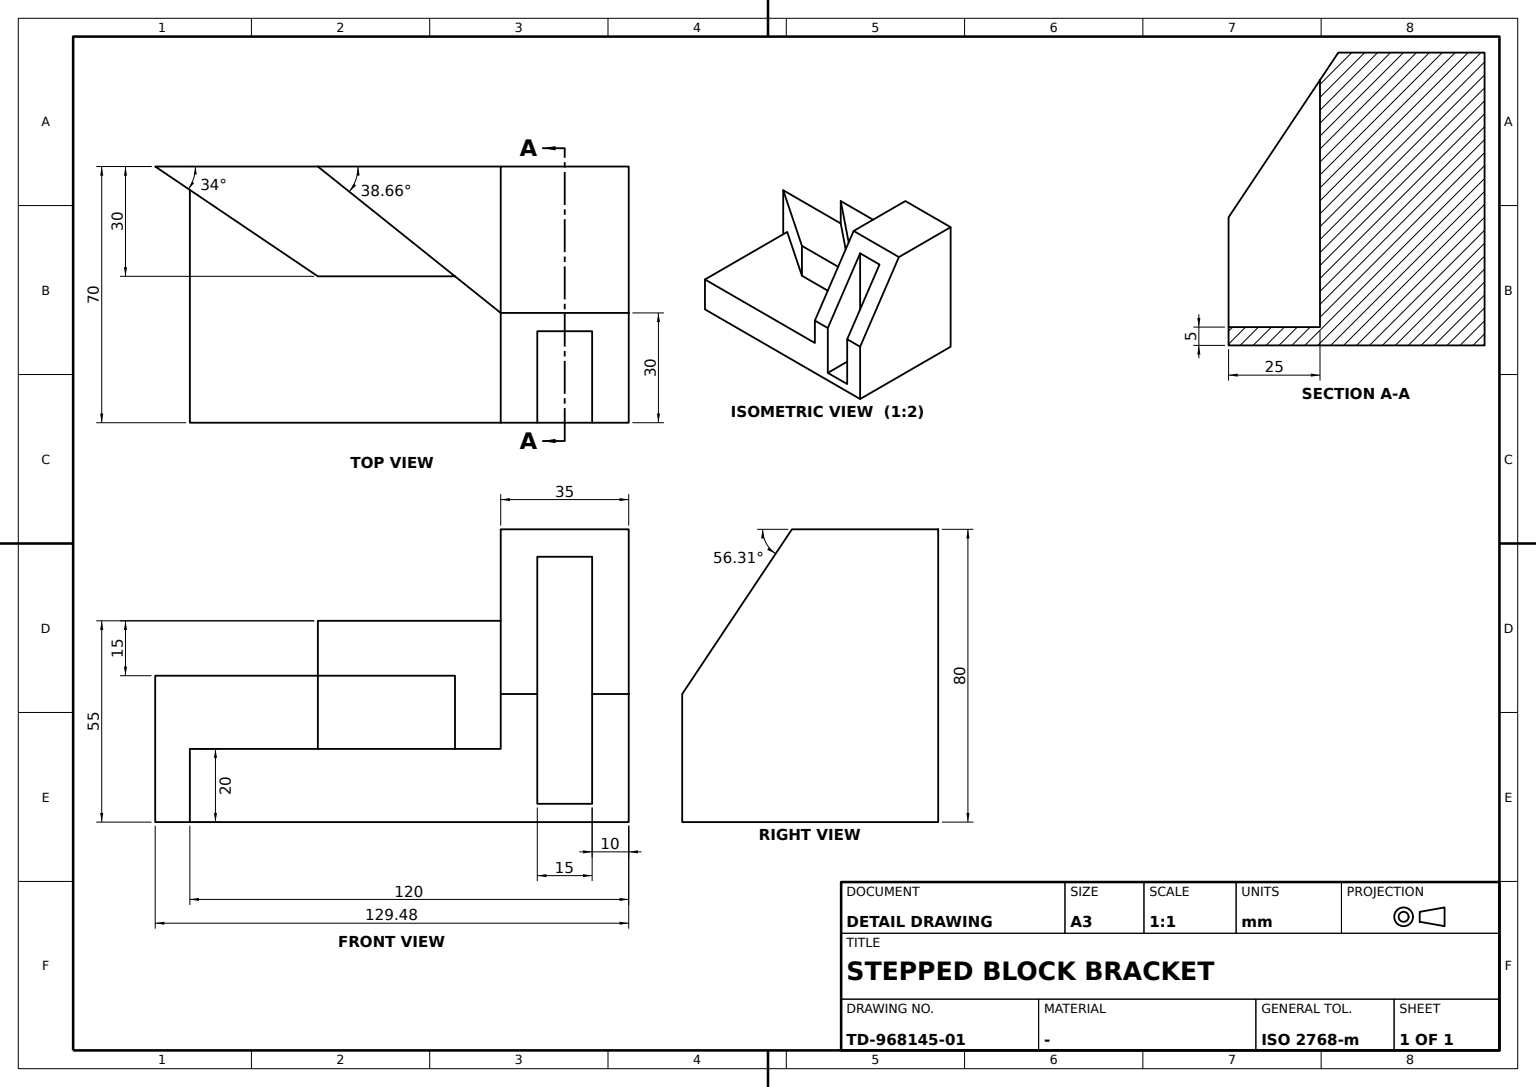
ISO-10303-21;
HEADER;
FILE_DESCRIPTION((''),'2;1');
FILE_NAME('','',(''),(''),'','','');
FILE_SCHEMA(('AUTOMOTIVE_DESIGN'));
ENDSEC;
DATA;
#1=APPLICATION_CONTEXT('');
#2=PRODUCT_CONTEXT('',#1,'mechanical');
#3=PRODUCT('','','',(#2));
#4=PRODUCT_DEFINITION_FORMATION('','',#3);
#5=PRODUCT_DEFINITION_CONTEXT('',#1,'design');
#6=PRODUCT_DEFINITION('','',#4,#5);
#7=PRODUCT_DEFINITION_SHAPE('','',#6);
#8=(LENGTH_UNIT()NAMED_UNIT(*)SI_UNIT(.MILLI.,.METRE.));
#9=(NAMED_UNIT(*)PLANE_ANGLE_UNIT()SI_UNIT($,.RADIAN.));
#10=(NAMED_UNIT(*)SI_UNIT($,.STERADIAN.)SOLID_ANGLE_UNIT());
#11=UNCERTAINTY_MEASURE_WITH_UNIT(LENGTH_MEASURE(0.005),#8,'distance_accuracy_value','');
#12=(GEOMETRIC_REPRESENTATION_CONTEXT(3)GLOBAL_UNCERTAINTY_ASSIGNED_CONTEXT((#11))GLOBAL_UNIT_ASSIGNED_CONTEXT((#8,#9,#10))REPRESENTATION_CONTEXT('',''));
#13=CARTESIAN_POINT('',(35.,50.,5.));
#14=VERTEX_POINT('',#13);
#15=CARTESIAN_POINT('',(35.,50.,35.));
#16=VERTEX_POINT('',#15);
#17=DIRECTION('',(0.,0.,1.));
#18=VECTOR('',#17,1000.);
#19=LINE('',#13,#18);
#20=EDGE_CURVE('',#14,#16,#19,.T.);
#21=ORIENTED_EDGE('',*,*,#20,.F.);
#22=CARTESIAN_POINT('',(35.,35.,5.));
#23=VERTEX_POINT('',#22);
#24=DIRECTION('',(0.,1.,0.));
#25=VECTOR('',#24,1000.);
#26=LINE('',#22,#25);
#27=EDGE_CURVE('',#23,#14,#26,.T.);
#28=ORIENTED_EDGE('',*,*,#27,.F.);
#29=CARTESIAN_POINT('',(35.,35.,35.));
#30=VERTEX_POINT('',#29);
#31=LINE('',#22,#18);
#32=EDGE_CURVE('',#23,#30,#31,.T.);
#33=ORIENTED_EDGE('',*,*,#32,.T.);
#34=CARTESIAN_POINT('',(35.,25.,35.));
#35=VERTEX_POINT('',#34);
#36=CARTESIAN_POINT('',(35.,85.,35.));
#37=DIRECTION('',(0.,-1.,0.));
#38=VECTOR('',#37,1000.);
#39=LINE('',#36,#38);
#40=EDGE_CURVE('',#30,#35,#39,.T.);
#41=ORIENTED_EDGE('',*,*,#40,.T.);
#42=CARTESIAN_POINT('',(35.,25.,20.));
#43=VERTEX_POINT('',#42);
#44=CARTESIAN_POINT('',(35.,25.,80.));
#45=DIRECTION('',(0.,0.,-1.));
#46=VECTOR('',#45,1000.);
#47=LINE('',#44,#46);
#48=EDGE_CURVE('',#35,#43,#47,.T.);
#49=ORIENTED_EDGE('',*,*,#48,.T.);
#50=CARTESIAN_POINT('',(35.,-60.,20.));
#51=VERTEX_POINT('',#50);
#52=LINE('',#50,#25);
#53=EDGE_CURVE('',#51,#43,#52,.T.);
#54=ORIENTED_EDGE('',*,*,#53,.F.);
#55=CARTESIAN_POINT('',(35.,-60.,0.));
#56=VERTEX_POINT('',#55);
#57=LINE('',#50,#46);
#58=EDGE_CURVE('',#51,#56,#57,.T.);
#59=ORIENTED_EDGE('',*,*,#58,.T.);
#60=CARTESIAN_POINT('',(35.,60.,0.));
#61=VERTEX_POINT('',#60);
#62=LINE('',#55,#25);
#63=EDGE_CURVE('',#56,#61,#62,.T.);
#64=ORIENTED_EDGE('',*,*,#63,.T.);
#65=CARTESIAN_POINT('',(35.,60.,35.));
#66=VERTEX_POINT('',#65);
#67=CARTESIAN_POINT('',(35.,60.,20.));
#68=LINE('',#67,#46);
#69=EDGE_CURVE('',#66,#61,#68,.T.);
#70=ORIENTED_EDGE('',*,*,#69,.F.);
#71=EDGE_CURVE('',#66,#16,#39,.T.);
#72=ORIENTED_EDGE('',*,*,#71,.T.);
#73=EDGE_LOOP('',(#21,#28,#33,#41,#49,#54,#59,#64,#70,#72));
#74=FACE_BOUND('',#73,.T.);
#75=DIRECTION('',(-1.,0.,0.));
#76=AXIS2_PLACEMENT_3D('',#50,#75,#37);
#77=PLANE('',#76);
#78=ADVANCED_FACE('',(#74),#77,.F.);
#79=CARTESIAN_POINT('',(5.,60.,80.));
#80=VERTEX_POINT('',#79);
#81=CARTESIAN_POINT('',(41.923077,60.,24.615385));
#82=DIRECTION('',(0.554700196,0.,-0.832050294));
#83=VECTOR('',#82,1000.);
#84=LINE('',#81,#83);
#85=EDGE_CURVE('',#80,#66,#84,.T.);
#86=ORIENTED_EDGE('',*,*,#85,.F.);
#87=CARTESIAN_POINT('',(5.,25.,80.));
#88=VERTEX_POINT('',#87);
#89=CARTESIAN_POINT('',(5.,85.,80.));
#90=LINE('',#89,#38);
#91=EDGE_CURVE('',#80,#88,#90,.T.);
#92=ORIENTED_EDGE('',*,*,#91,.T.);
#93=LINE('',#87,#83);
#94=EDGE_CURVE('',#88,#35,#93,.T.);
#95=ORIENTED_EDGE('',*,*,#94,.T.);
#96=ORIENTED_EDGE('',*,*,#40,.F.);
#97=CARTESIAN_POINT('',(10.,35.,72.5));
#98=VERTEX_POINT('',#97);
#99=CARTESIAN_POINT('',(5.,35.,80.));
#100=DIRECTION('',(-0.554700196,0.,0.832050294));
#101=VECTOR('',#100,1000.);
#102=LINE('',#99,#101);
#103=EDGE_CURVE('',#30,#98,#102,.T.);
#104=ORIENTED_EDGE('',*,*,#103,.T.);
#105=CARTESIAN_POINT('',(10.,50.,72.5));
#106=VERTEX_POINT('',#105);
#107=CARTESIAN_POINT('',(10.,85.,72.5));
#108=LINE('',#107,#25);
#109=EDGE_CURVE('',#98,#106,#108,.T.);
#110=ORIENTED_EDGE('',*,*,#109,.T.);
#111=CARTESIAN_POINT('',(5.,50.,80.));
#112=LINE('',#111,#83);
#113=EDGE_CURVE('',#106,#16,#112,.T.);
#114=ORIENTED_EDGE('',*,*,#113,.T.);
#115=ORIENTED_EDGE('',*,*,#71,.F.);
#116=EDGE_LOOP('',(#86,#92,#95,#96,#104,#110,#114,#115));
#117=FACE_BOUND('',#116,.T.);
#118=DIRECTION('',(-0.832050294,0.,-0.554700196));
#119=AXIS2_PLACEMENT_3D('',#89,#118,#100);
#120=PLANE('',#119);
#121=ADVANCED_FACE('',(#117),#120,.F.);
#122=CARTESIAN_POINT('',(10.,35.,5.));
#123=VERTEX_POINT('',#122);
#124=VECTOR('',#75,1000.);
#125=LINE('',#122,#124);
#126=EDGE_CURVE('',#23,#123,#125,.T.);
#127=ORIENTED_EDGE('',*,*,#126,.T.);
#128=LINE('',#122,#46);
#129=EDGE_CURVE('',#98,#123,#128,.T.);
#130=ORIENTED_EDGE('',*,*,#129,.F.);
#131=ORIENTED_EDGE('',*,*,#103,.F.);
#132=ORIENTED_EDGE('',*,*,#32,.F.);
#133=EDGE_LOOP('',(#127,#130,#131,#132));
#134=FACE_BOUND('',#133,.T.);
#135=AXIS2_PLACEMENT_3D('',#122,#37,#45);
#136=PLANE('',#135);
#137=ADVANCED_FACE('',(#134),#136,.F.);
#138=CARTESIAN_POINT('',(-35.,-25.,40.));
#139=VERTEX_POINT('',#138);
#140=CARTESIAN_POINT('',(-5.,12.5,40.));
#141=VERTEX_POINT('',#140);
#142=DIRECTION('',(0.624695048,0.780868809,0.));
#143=VECTOR('',#142,1000.);
#144=LINE('',#138,#143);
#145=EDGE_CURVE('',#139,#141,#144,.T.);
#146=ORIENTED_EDGE('',*,*,#145,.F.);
#147=CARTESIAN_POINT('',(-35.,-69.476829,40.));
#148=VERTEX_POINT('',#147);
#149=LINE('',#147,#25);
#150=EDGE_CURVE('',#148,#139,#149,.T.);
#151=ORIENTED_EDGE('',*,*,#150,.F.);
#152=CARTESIAN_POINT('',(-5.,-25.,40.));
#153=VERTEX_POINT('',#152);
#154=DIRECTION('',(-0.559192903,-0.829037573,0.));
#155=VECTOR('',#154,1000.);
#156=LINE('',#152,#155);
#157=EDGE_CURVE('',#153,#148,#156,.T.);
#158=ORIENTED_EDGE('',*,*,#157,.F.);
#159=LINE('',#140,#38);
#160=EDGE_CURVE('',#141,#153,#159,.T.);
#161=ORIENTED_EDGE('',*,*,#160,.F.);
#162=EDGE_LOOP('',(#146,#151,#158,#161));
#163=FACE_BOUND('',#162,.T.);
#164=CARTESIAN_POINT('',(0.,0.,40.));
#165=AXIS2_PLACEMENT_3D('',#164,#45,#75);
#166=PLANE('',#165);
#167=ADVANCED_FACE('',(#163),#166,.F.);
#168=CARTESIAN_POINT('',(-35.,25.,80.));
#169=VERTEX_POINT('',#168);
#170=DIRECTION('',(1.,0.,0.));
#171=VECTOR('',#170,1000.);
#172=LINE('',#168,#171);
#173=EDGE_CURVE('',#169,#88,#172,.T.);
#174=ORIENTED_EDGE('',*,*,#173,.F.);
#175=CARTESIAN_POINT('',(-35.,25.,55.));
#176=VERTEX_POINT('',#175);
#177=LINE('',#168,#46);
#178=EDGE_CURVE('',#169,#176,#177,.T.);
#179=ORIENTED_EDGE('',*,*,#178,.T.);
#180=CARTESIAN_POINT('',(5.,25.,55.));
#181=VERTEX_POINT('',#180);
#182=LINE('',#180,#124);
#183=EDGE_CURVE('',#181,#176,#182,.T.);
#184=ORIENTED_EDGE('',*,*,#183,.F.);
#185=CARTESIAN_POINT('',(5.,25.,20.));
#186=VERTEX_POINT('',#185);
#187=LINE('',#180,#46);
#188=EDGE_CURVE('',#181,#186,#187,.T.);
#189=ORIENTED_EDGE('',*,*,#188,.T.);
#190=CARTESIAN_POINT('',(-35.,25.,20.));
#191=LINE('',#190,#171);
#192=EDGE_CURVE('',#186,#43,#191,.T.);
#193=ORIENTED_EDGE('',*,*,#192,.T.);
#194=ORIENTED_EDGE('',*,*,#48,.F.);
#195=ORIENTED_EDGE('',*,*,#94,.F.);
#196=EDGE_LOOP('',(#174,#179,#184,#189,#193,#194,#195));
#197=FACE_BOUND('',#196,.T.);
#198=AXIS2_PLACEMENT_3D('',#168,#24,#75);
#199=PLANE('',#198);
#200=ADVANCED_FACE('',(#197),#199,.F.);
#201=CARTESIAN_POINT('',(-35.,60.,0.));
#202=VERTEX_POINT('',#201);
#203=LINE('',#60,#124);
#204=EDGE_CURVE('',#61,#202,#203,.T.);
#205=ORIENTED_EDGE('',*,*,#204,.F.);
#206=ORIENTED_EDGE('',*,*,#63,.F.);
#207=CARTESIAN_POINT('',(-28.607798,-60.,0.));
#208=VERTEX_POINT('',#207);
#209=CARTESIAN_POINT('',(-35.,-60.,0.));
#210=LINE('',#209,#171);
#211=EDGE_CURVE('',#208,#56,#210,.T.);
#212=ORIENTED_EDGE('',*,*,#211,.F.);
#213=CARTESIAN_POINT('',(-35.,-69.476829,0.));
#214=VERTEX_POINT('',#213);
#215=CARTESIAN_POINT('',(-5.,-25.,0.));
#216=LINE('',#215,#155);
#217=EDGE_CURVE('',#208,#214,#216,.T.);
#218=ORIENTED_EDGE('',*,*,#217,.T.);
#219=LINE('',#201,#38);
#220=EDGE_CURVE('',#202,#214,#219,.T.);
#221=ORIENTED_EDGE('',*,*,#220,.F.);
#222=EDGE_LOOP('',(#205,#206,#212,#218,#221));
#223=FACE_BOUND('',#222,.T.);
#224=CARTESIAN_POINT('',(0.,0.,0.));
#225=AXIS2_PLACEMENT_3D('',#224,#17,#170);
#226=PLANE('',#225);
#227=ADVANCED_FACE('',(#223),#226,.F.);
#228=ORIENTED_EDGE('',*,*,#150,.T.);
#229=CARTESIAN_POINT('',(-35.,-25.,55.));
#230=VERTEX_POINT('',#229);
#231=LINE('',#229,#46);
#232=EDGE_CURVE('',#230,#139,#231,.T.);
#233=ORIENTED_EDGE('',*,*,#232,.F.);
#234=LINE('',#175,#38);
#235=EDGE_CURVE('',#176,#230,#234,.T.);
#236=ORIENTED_EDGE('',*,*,#235,.F.);
#237=ORIENTED_EDGE('',*,*,#178,.F.);
#238=CARTESIAN_POINT('',(-35.,60.,80.));
#239=VERTEX_POINT('',#238);
#240=LINE('',#238,#38);
#241=EDGE_CURVE('',#239,#169,#240,.T.);
#242=ORIENTED_EDGE('',*,*,#241,.F.);
#243=CARTESIAN_POINT('',(-35.,60.,20.));
#244=LINE('',#243,#46);
#245=EDGE_CURVE('',#239,#202,#244,.T.);
#246=ORIENTED_EDGE('',*,*,#245,.T.);
#247=ORIENTED_EDGE('',*,*,#220,.T.);
#248=LINE('',#147,#46);
#249=EDGE_CURVE('',#148,#214,#248,.T.);
#250=ORIENTED_EDGE('',*,*,#249,.F.);
#251=EDGE_LOOP('',(#228,#233,#236,#237,#242,#246,#247,#250));
#252=FACE_BOUND('',#251,.T.);
#253=AXIS2_PLACEMENT_3D('',#243,#170,#24);
#254=PLANE('',#253);
#255=ADVANCED_FACE('',(#252),#254,.F.);
#256=ORIENTED_EDGE('',*,*,#58,.F.);
#257=CARTESIAN_POINT('',(-28.607798,-60.,20.));
#258=VERTEX_POINT('',#257);
#259=CARTESIAN_POINT('',(-35.,-60.,20.));
#260=LINE('',#259,#171);
#261=EDGE_CURVE('',#258,#51,#260,.T.);
#262=ORIENTED_EDGE('',*,*,#261,.F.);
#263=LINE('',#257,#46);
#264=EDGE_CURVE('',#258,#208,#263,.T.);
#265=ORIENTED_EDGE('',*,*,#264,.T.);
#266=ORIENTED_EDGE('',*,*,#211,.T.);
#267=EDGE_LOOP('',(#256,#262,#265,#266));
#268=FACE_BOUND('',#267,.T.);
#269=AXIS2_PLACEMENT_3D('',#259,#24,#75);
#270=PLANE('',#269);
#271=ADVANCED_FACE('',(#268),#270,.F.);
#272=ORIENTED_EDGE('',*,*,#241,.T.);
#273=ORIENTED_EDGE('',*,*,#173,.T.);
#274=ORIENTED_EDGE('',*,*,#91,.F.);
#275=CARTESIAN_POINT('',(35.,60.,80.));
#276=LINE('',#275,#124);
#277=EDGE_CURVE('',#80,#239,#276,.T.);
#278=ORIENTED_EDGE('',*,*,#277,.T.);
#279=EDGE_LOOP('',(#272,#273,#274,#278));
#280=FACE_BOUND('',#279,.T.);
#281=CARTESIAN_POINT('',(0.,0.,80.));
#282=AXIS2_PLACEMENT_3D('',#281,#17,#170);
#283=PLANE('',#282);
#284=ADVANCED_FACE('',(#280),#283,.T.);
#285=CARTESIAN_POINT('',(10.,50.,5.));
#286=VERTEX_POINT('',#285);
#287=LINE('',#285,#25);
#288=EDGE_CURVE('',#123,#286,#287,.T.);
#289=ORIENTED_EDGE('',*,*,#288,.T.);
#290=LINE('',#285,#46);
#291=EDGE_CURVE('',#106,#286,#290,.T.);
#292=ORIENTED_EDGE('',*,*,#291,.F.);
#293=ORIENTED_EDGE('',*,*,#109,.F.);
#294=ORIENTED_EDGE('',*,*,#129,.T.);
#295=EDGE_LOOP('',(#289,#292,#293,#294));
#296=FACE_BOUND('',#295,.T.);
#297=AXIS2_PLACEMENT_3D('',#285,#75,#37);
#298=PLANE('',#297);
#299=ADVANCED_FACE('',(#296),#298,.F.);
#300=ORIENTED_EDGE('',*,*,#249,.T.);
#301=ORIENTED_EDGE('',*,*,#217,.F.);
#302=ORIENTED_EDGE('',*,*,#264,.F.);
#303=CARTESIAN_POINT('',(-5.,-25.,20.));
#304=VERTEX_POINT('',#303);
#305=CARTESIAN_POINT('',(8.153282,-5.499458,20.));
#306=DIRECTION('',(0.559192903,0.829037573,0.));
#307=VECTOR('',#306,1000.);
#308=LINE('',#305,#307);
#309=EDGE_CURVE('',#258,#304,#308,.T.);
#310=ORIENTED_EDGE('',*,*,#309,.T.);
#311=LINE('',#152,#46);
#312=EDGE_CURVE('',#153,#304,#311,.T.);
#313=ORIENTED_EDGE('',*,*,#312,.F.);
#314=ORIENTED_EDGE('',*,*,#157,.T.);
#315=EDGE_LOOP('',(#300,#301,#302,#310,#313,#314));
#316=FACE_BOUND('',#315,.T.);
#317=DIRECTION('',(0.829037573,-0.559192903,0.));
#318=AXIS2_PLACEMENT_3D('',#152,#317,#306);
#319=PLANE('',#318);
#320=ADVANCED_FACE('',(#316),#319,.T.);
#321=ORIENTED_EDGE('',*,*,#291,.T.);
#322=LINE('',#13,#171);
#323=EDGE_CURVE('',#286,#14,#322,.T.);
#324=ORIENTED_EDGE('',*,*,#323,.T.);
#325=ORIENTED_EDGE('',*,*,#20,.T.);
#326=ORIENTED_EDGE('',*,*,#113,.F.);
#327=EDGE_LOOP('',(#321,#324,#325,#326));
#328=FACE_BOUND('',#327,.T.);
#329=AXIS2_PLACEMENT_3D('',#13,#24,#17);
#330=PLANE('',#329);
#331=ADVANCED_FACE('',(#328),#330,.F.);
#332=ORIENTED_EDGE('',*,*,#235,.T.);
#333=LINE('',#229,#143);
#334=EDGE_CURVE('',#230,#181,#333,.T.);
#335=ORIENTED_EDGE('',*,*,#334,.T.);
#336=ORIENTED_EDGE('',*,*,#183,.T.);
#337=EDGE_LOOP('',(#332,#335,#336));
#338=FACE_BOUND('',#337,.T.);
#339=CARTESIAN_POINT('',(0.,0.,55.));
#340=AXIS2_PLACEMENT_3D('',#339,#45,#75);
#341=PLANE('',#340);
#342=ADVANCED_FACE('',(#338),#341,.F.);
#343=ORIENTED_EDGE('',*,*,#204,.T.);
#344=ORIENTED_EDGE('',*,*,#245,.F.);
#345=ORIENTED_EDGE('',*,*,#277,.F.);
#346=ORIENTED_EDGE('',*,*,#85,.T.);
#347=ORIENTED_EDGE('',*,*,#69,.T.);
#348=EDGE_LOOP('',(#343,#344,#345,#346,#347));
#349=FACE_BOUND('',#348,.T.);
#350=AXIS2_PLACEMENT_3D('',#67,#37,#170);
#351=PLANE('',#350);
#352=ADVANCED_FACE('',(#349),#351,.F.);
#353=CARTESIAN_POINT('',(-5.,12.5,20.));
#354=VERTEX_POINT('',#353);
#355=CARTESIAN_POINT('',(-5.,0.,20.));
#356=LINE('',#355,#25);
#357=EDGE_CURVE('',#304,#354,#356,.T.);
#358=ORIENTED_EDGE('',*,*,#357,.T.);
#359=LINE('',#140,#46);
#360=EDGE_CURVE('',#141,#354,#359,.T.);
#361=ORIENTED_EDGE('',*,*,#360,.F.);
#362=ORIENTED_EDGE('',*,*,#160,.T.);
#363=ORIENTED_EDGE('',*,*,#312,.T.);
#364=EDGE_LOOP('',(#358,#361,#362,#363));
#365=FACE_BOUND('',#364,.T.);
#366=AXIS2_PLACEMENT_3D('',#140,#170,#24);
#367=PLANE('',#366);
#368=ADVANCED_FACE('',(#365),#367,.T.);
#369=ORIENTED_EDGE('',*,*,#323,.F.);
#370=ORIENTED_EDGE('',*,*,#288,.F.);
#371=ORIENTED_EDGE('',*,*,#126,.F.);
#372=ORIENTED_EDGE('',*,*,#27,.T.);
#373=EDGE_LOOP('',(#369,#370,#371,#372));
#374=FACE_BOUND('',#373,.T.);
#375=CARTESIAN_POINT('',(0.,0.,5.));
#376=AXIS2_PLACEMENT_3D('',#375,#17,#170);
#377=PLANE('',#376);
#378=ADVANCED_FACE('',(#374),#377,.T.);
#379=CARTESIAN_POINT('',(-35.,-25.,20.));
#380=LINE('',#379,#143);
#381=EDGE_CURVE('',#354,#186,#380,.T.);
#382=ORIENTED_EDGE('',*,*,#381,.T.);
#383=ORIENTED_EDGE('',*,*,#188,.F.);
#384=ORIENTED_EDGE('',*,*,#334,.F.);
#385=ORIENTED_EDGE('',*,*,#232,.T.);
#386=ORIENTED_EDGE('',*,*,#145,.T.);
#387=ORIENTED_EDGE('',*,*,#360,.T.);
#388=EDGE_LOOP('',(#382,#383,#384,#385,#386,#387));
#389=FACE_BOUND('',#388,.T.);
#390=DIRECTION('',(-0.780868809,0.624695048,0.));
#391=DIRECTION('',(-0.624695048,-0.780868809,0.));
#392=AXIS2_PLACEMENT_3D('',#229,#390,#391);
#393=PLANE('',#392);
#394=ADVANCED_FACE('',(#389),#393,.F.);
#395=ORIENTED_EDGE('',*,*,#357,.F.);
#396=ORIENTED_EDGE('',*,*,#309,.F.);
#397=ORIENTED_EDGE('',*,*,#261,.T.);
#398=ORIENTED_EDGE('',*,*,#53,.T.);
#399=ORIENTED_EDGE('',*,*,#192,.F.);
#400=ORIENTED_EDGE('',*,*,#381,.F.);
#401=EDGE_LOOP('',(#395,#396,#397,#398,#399,#400));
#402=FACE_BOUND('',#401,.T.);
#403=CARTESIAN_POINT('',(0.,0.,20.));
#404=AXIS2_PLACEMENT_3D('',#403,#17,#170);
#405=PLANE('',#404);
#406=ADVANCED_FACE('',(#402),#405,.T.);
#407=CLOSED_SHELL('',(#78,#121,#137,#167,#200,#227,#255,#271,#284,#299,#320,#331,#342,#352,#368,#378,#394,#406));
#408=MANIFOLD_SOLID_BREP('',#407);
#409=ADVANCED_BREP_SHAPE_REPRESENTATION('',(#408),#12);
#410=SHAPE_DEFINITION_REPRESENTATION(#7,#409);
ENDSEC;
END-ISO-10303-21;
